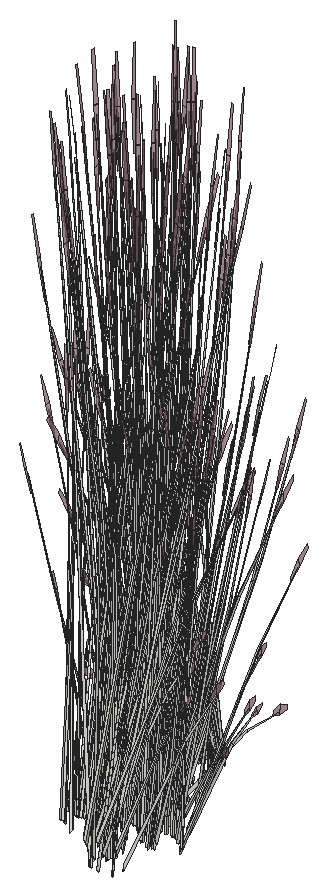
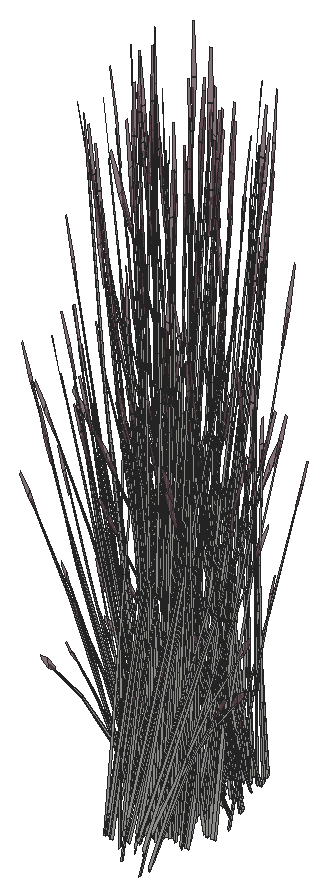
# SketchUp Ruby script. Lengths in inches.
U = 1.inch
M = Sketchup.active_model
def pt(a) = Geom::Point3d.new(a.map { |v| v * U })
def face(e, loops, mat)
  f = e.add_face(loops[0].map { |a| pt(a) })
  loops[1..].each { |l| e.add_face(l.map { |a| pt(a) }).erase! }
  f.material = f.back_material = mat if mat
  f
end
# faces: each face lists its corners as indices into pts; further lists are holes
def faces(e, pts, list, mat = nil) = list.each { |f| face(e, (f[0].is_a?(Array) ? f : [f]).map { |l| l.map { |i| pts[i] } }, mat) }
# xy, xz, yz: faces in a plane at the given z, y or x. An outline is a flat list of corners, or four numbers for a rectangle; further outlines are holes
def ring(l) = l.size == 4 ? [[l[0], l[1]], [l[2], l[1]], [l[2], l[3]], [l[0], l[3]]] : l.each_slice(2).to_a
def flat(e, list, mat, &to3) = list.each { |f| face(e, (f[0].is_a?(Array) ? f : [f]).map { |l| ring(l).map { |u, v| to3.(u, v) } }, mat) }
def xy(e, z, list, mat = nil) = flat(e, list, mat) { |x, y| [x, y, z] }
def xz(e, y, list, mat = nil) = flat(e, list, mat) { |x, z| [x, y, z] }
def yz(e, x, list, mat = nil) = flat(e, list, mat) { |y, z| [x, y, z] }
def lines(e, pts, list) = list.each { |a, b| e.add_line(pt(pts[a]), pt(pts[b])) }
# prism: a flat outline (further loops are holes) pulled along v
def prism(e, loops, v, mat = nil)
  f = face(e, loops, mat); d = Geom::Vector3d.new(v.map { |x| x * U })
  f.pushpull(f.normal.samedirection?(d) ? d.length : -d.length)
end
def box(e, o, s, mat = nil) = prism(e, [[o, [o[0] + s[0], o[1], o[2]], [o[0] + s[0], o[1] + s[1], o[2]], [o[0], o[1] + s[1], o[2]]]], [0, 0, s[2]], mat)
def at(x, y, z, deg = 0) = Geom::Transformation.translation(pt([x, y, z])) * Geom::Transformation.rotation(ORIGIN, Z_AXIS, deg.degrees)
def axes(o, x, y, z) = Geom::Transformation.new([*x, 0, *y, 0, *z, 0, *pt(o).to_a, 1])
def part(name) = M.definitions.add(name)
# library, detail: a bought-in or finely detailed component or shape, given as its bounding box
def library(name, o, s) = part(name).tap { |d| box(d.entities, o, s) }
def detail(e, o, s) = box(e.add_group.entities, o, s)
def put(e, d, t, mat = nil) = e.add_instance(d, t).tap { |i| i.material = mat if mat }
def group(e, t, mat = nil) = e.add_group.tap { |g| g.transformation = t; g.material = mat if mat }.entities
root = M.entities
M.materials.add("LightPink_Translucent").color = [144, 107, 117]
M.materials["LightPink_Translucent"].alpha = 0.75
c1 = part("blade")
p = [[2.15,0.21,22],[0,0.17,0],[0.09,0.45,0],[2.18,0.31,22],[2.29,0.31,22],[0.38,0.45,0],
  [2.48,0.24,33],[2.49,0.24,33],[2.48,0.22,33]]
faces(c1.entities,p,[[0,1,2,3],[4,5,2,3],[6,3,4,7],[8,0,3,6]])
c2 = part("seeds")
p = [[0.3,-0.1,1.38],[-0.01,-0.03,1.59],[-0.01,-0.03,0.03],[0.14,-0.07,-0.07],[0.29,-0.03,3],[0.15,0.01,3.11]]
faces(c2.entities,p,[[0,1,2,3],[1,0,4,5]],"LightPink_Translucent")
c3 = part("blade with seeds")
put(c3.entities,c1,at(0,0,0))
put(c3.entities,c2,axes([2.4,0.25,30.99],[1.5799,-0.05474,1.17369],[-0.12525,1.92788,0.29478],[-0.07173,-0.02425,1.56792]))
put(root,c3,axes([411.74,290.53,-9.94],[-0.24813,0.48978,-0.41661],[-0.51557,-0.23571,0.2005],[0,0.1129,1.33761]))
put(root,c3,axes([412.8,291.68,-7.59],[-0.37709,0.35815,0.447],[-0.32522,-0.38035,0.36857],[0.17692,0.06607,0.92496]))
put(root,c3,axes([411.27,295.7,-10.08],[0.34446,-0.40855,-0.58063],[0.42791,0.37046,-0.15239],[0.13803,-0.10191,1.28164]))
put(root,c3,axes([413.76,294.73,-9.42],[-0.17034,0.27669,1.06958],[-0.14642,-0.37174,0.78586],[0.14069,-0.09315,0.23558]))
put(root,c3,axes([413.51,295.77,-7.78],[0.44516,-0.07768,-0.32977],[0.11755,0.44407,0.42575],[0.12757,-0.11927,0.81462]))
put(root,c3,axes([407.94,292.07,-6.74],[0.45129,0.14509,-0.06041],[-0.13882,0.44656,-0.27392],[-0.07381,0.0678,0.90349]))
put(root,c3,axes([411.14,291.24,-10.08],[-0.34446,0.40855,-0.58063],[-0.42791,-0.37046,-0.15239],[-0.13803,0.10191,1.28164]))
put(root,c3,axes([409.34,295.03,-7.6],[0.02575,-0.41332,0.05988],[0.38885,0.01133,0.47138],[-0.14895,-0.04325,0.71878]))
put(root,c3,axes([411.6,292.1,-7.3],[-0.07899,-0.43781,0.32977],[0.45153,-0.11561,-0.42575],[0.12128,0.12546,0.81462]))
put(root,c3,axes([410.67,296.42,-9.94],[0.24813,-0.48978,-0.41661],[0.51557,0.23571,0.2005],[0,-0.1129,1.33761]))
put(root,c3,axes([411.76,291.93,-9.83],[0.64025,0.17667,0.2864],[-0.16018,0.63149,-0.33981],[-0.10597,0.07904,1.53541]))
put(root,c3,axes([411.71,292.36,-10.12],[-0.47863,0.27177,-0.46235],[-0.28609,-0.48733,0],[-0.10901,0.0619,1.46668]))
put(root,c3,axes([413.3,290.75,-10.12],[0,0.54355,-0.46235],[-0.57217,0,0],[0,0.1238,1.46668]))
put(root,c3,axes([410.9,296.17,-9.52],[-0.05959,-0.62022,-0.27094],[0.62068,-0.0375,-0.46562],[0.1093,-0.08261,1.4872]))
put(root,c3,axes([411.87,290.81,-8.39],[-0.18996,-0.09365,1.59586],[0.39312,-0.39287,0.12904],[0.24502,0.17723,0.68222]))
put(root,c3,axes([409.36,296.21,-10.11],[0.35699,-0.33913,-0.28847],[0.35699,0.33913,0.28847],[0,-0.10923,1.29413]))
put(root,c3,axes([411.91,289.58,-7.83],[-0.44191,-0.28242,1.28769],[0.46662,-0.43971,0.5556],[0.14258,0.26499,1.24467]))
put(root,c3,axes([409.22,294.58,-10.02],[-0.14753,0.44383,-0.03625],[-0.45406,-0.13653,-0.16435],[-0.06894,-0.07259,0.54209]))
put(root,c3,axes([413.15,296.03,-7.3],[-0.44516,0.07768,0.32977],[-0.11755,-0.44407,-0.42575],[0.12757,-0.11927,0.81462]))
put(root,c3,axes([410.61,296.82,-9.52],[-0.57594,-0.25935,-0.27094],[0.27732,-0.5474,-0.46562],[-0.0181,-0.1344,1.4872]))
put(root,c3,axes([408.97,296.61,-9.79],[-0.63949,0,0],[0,-0.60749,-0.48057],[0,-0.13836,1.52448]))
put(root,c3,axes([408.72,290.77,-7.3125],[0.47307,0.29971,-0.11324],[-0.27254,0.43404,-0.62851],[-0.13365,0.15087,0.95501]))
put(root,c3,axes([412.57,291.875,-9.42],[-0.28795,-0.15629,1.06958],[0.37181,-0.1588,0.78586],[0.10029,0.13452,0.23558]))
put(root,c3,axes([411.5625,292.32,-7.3125],[0.30474,-0.46525,-0.11324],[0.44133,0.26804,-0.62851],[0.15341,0.13145,0.95501]))
put(root,c3,axes([410.82,294.8,-10.11],[0.47712,0.13449,-0.28847],[-0.12013,0.47362,0.28847],[0.09619,-0.05462,1.29413]))
put(root,c3,axes([408.95,291.125,-7.64],[0.13138,0.49631,-0.47583],[-0.49754,0.08682,-0.36857],[-0.14258,0.13331,0.91046]))
put(root,c3,axes([409.55,291.69,-7.3],[0.34603,-0.28618,0.32977],[0.32756,0.32677,-0.42575],[-0.04984,0.16603,0.81462]))
put(root,c3,axes([412.14,292.27,-9.79],[0.31974,0.54466,0],[-0.53494,0.30375,-0.48057],[-0.12184,0.06918,1.52448]))
put(root,c3,axes([411.16,292.71,-7.62],[0.00151,-0.06581,1.65179],[0.43826,-0.29033,-0.15608],[0.15223,0.10363,0.29231]))
put(root,c3,axes([413.55,295.96,-7.6],[0.35109,0.22859,0.05988],[-0.2044,0.32553,0.47138],[0.11256,-0.10524,0.71878]))
put(root,c3,axes([412.65,292.46,-10.61],[0.03726,-0.07847,1.6421],[0.46909,-0.23111,-0.25086],[0.14221,0.11962,0.2797]))
put(root,c3,axes([413.46,295.87,-7.59],[0.12683,0.50025,0.447],[-0.49754,0.08682,0.36857],[0.14663,-0.11765,0.92496]))
put(root,c3,axes([411.87,290.12,-9.35],[-0.01397,-0.51177,1.31553],[0.63227,0.13266,0.557],[-0.14954,0.28003,1.24175]))
put(root,c3,axes([412.03,290.67,-10.05],[0.18752,0.49766,-0.6445],[-0.54017,0.17923,-0.16915],[0.02073,0.16852,1.42262]))
put(root,c3,axes([409.24,291.95,-7.6],[-0.42027,-0.02533,0.05988],[0.01152,-0.38243,0.47138],[-0.04398,0.14649,0.71878]))
put(root,c3,axes([414.8,296.47,-7.61],[0.07097,-0.08279,1.62908],[-0.09083,-0.50786,-0.25764],[0.17806,-0.09629,0.13065]))
put(root,c3,axes([409.37,291.99,-7.59],[-0.36417,-0.37086,0.447],[0.38674,-0.31985,0.36857],[-0.06718,0.174,0.92496]))
put(root,c3,axes([411.92,292.09,-7.64],[0.50465,-0.12921,-0.47583],[0.08828,0.48932,-0.36857],[0.13555,0.14022,0.91046]))
put(root,c3,axes([410.52,292.16,-7.3],[0.15418,-0.41799,0.32977],[0.44981,0.12192,-0.42575],[0.04124,0.16829,0.81462]))
put(root,c3,axes([409.47,296.45,-9.83],[-0.47569,0.45698,0.2864],[-0.47598,-0.45217,-0.33981],[-0.01661,-0.12977,1.53541]))
put(root,c3,axes([412.62,292.59,-9.52],[-0.32795,-0.01705,0.97832],[0.21658,-0.36206,0.54015],[0.12956,0.12863,0.76741]))
put(root,c3,axes([410.98,296.66,-9.73],[0.57623,0.26344,0.22409],[-0.27732,0.5474,0.46562],[0,-0.12618,1.49497]))
put(root,c3,axes([410.76,297.4,-9.73],[0.13555,-0.64407,-0.21817],[0.64269,0.11227,0.47743],[-0.1123,-0.08895,1.45677]))
put(root,c3,axes([411.67,292.49,-7.6],[-0.23243,0.34529,0.05988],[-0.331,-0.20103,0.47138],[0.10701,0.1107,0.71878]))
put(root,c3,axes([409.6,295.34,-7.3],[0.29098,0.34031,0.32977],[-0.33226,0.32215,-0.42575],[-0.16881,-0.04902,0.81462]))
put(root,c3,axes([411.13,293.66,-6.74],[0.35341,-0.31182,-0.06041],[0.32382,0.34152,-0.27392],[0.0228,0.09677,0.90349]))
put(root,c3,axes([411.77,292.4,-7.59],[-0.50866,0.12474,0.447],[-0.08828,-0.48932,0.36857],[0.11963,0.14421,0.92496]))
put(root,c3,axes([410.79,296.29,-9.47],[-0.55535,0.03355,0.41661],[-0.05022,-0.55698,-0.2005],[0.09942,-0.05645,1.33761]))
put(root,c3,axes([409.26,291.05,-8.39],[0.09522,-0.18683,1.59586],[0.39947,0.38663,0.12904],[-0.18021,0.24097,0.68222]))
put(root,c3,axes([409.36,296.7,-9.69],[0,0.54355,0.46235],[-0.57217,0,0],[0,-0.1238,1.46668]))
put(root,c3,axes([413.4,297.24,-7.3125],[-0.25732,-0.49218,-0.11324],[0.45669,-0.24187,-0.62851],[0.19245,-0.06494,0.95501]))
put(root,c3,axes([411.55,291.71,-9.59],[0.00902,-0.18018,1.33163],[0.43127,-0.20126,-0.28638],[0.13313,0.21566,0.56934]))
put(root,c3,axes([413.38,296.82,-7.64],[0.13855,-0.49442,-0.47583],[0.47502,0.16947,-0.36857],[0.19125,-0.04534,0.91046]))
put(root,c3,axes([412.625,294.81,-9.79],[0.31974,-0.54466,0],[0.53494,0.30375,-0.48057],[0.12184,0.06918,1.52448]))
put(root,c3,axes([410.71,297.14,-9.94],[-0.30722,-0.45622,-0.41661],[0.46535,-0.32126,0.2005],[-0.09942,-0.05645,1.33761]))
put(root,c3,axes([410.78,296.49,-9.8],[0.22235,0.6078,0.42607],[-0.63531,0.21135,0.16719],[0.00776,-0.11168,1.47927]))
put(root,c3,axes([410.38,292.54,-7.6],[-0.37684,0.18473,0.05988],[-0.18445,-0.33686,0.47138],[0.03639,0.14849,0.71878]))
put(root,c3,axes([409.37,292.1,-7.78],[-0.34603,0.28618,-0.32977],[-0.32756,-0.32677,0.42575],[-0.04984,0.16603,0.81462]))
put(root,c3,axes([408.18,292.02,-7.61],[-0.01271,0.10756,1.62908],[0.36076,0.37419,-0.25764],[-0.09444,0.17695,0.13065]))
put(root,c3,axes([409.33,291.77,-6.97],[0.56206,0.02693,-0.12569],[-0.01536,0.50991,-0.69765],[-0.03904,0.19638,1.06006]))
put(root,c3,axes([410.37,292.34,-7.3125],[0.50045,-0.25306,-0.11324],[0.24593,0.44915,-0.62851],[0.06603,0.18927,0.95501]))
put(root,c3,axes([413.88,296.96,-10.15],[-0.32938,0.06523,1.31842],[-0.05243,-0.51922,0.07547],[0.2307,-0.07859,0.75023]))
put(root,c3,axes([414.48,296.5,-9.89],[-0.31706,-0.34757,-0.06041],[0.34725,-0.31847,-0.27392],[0.09839,-0.02242,0.90349]))
put(root,c3,axes([410.52,292.51,-7.28],[-0.50393,-0.1421,0.49617],[0.17232,-0.46717,0.40911],[0.03028,0.18372,1.0267]))
put(root,c3,axes([409.59,293.21,-9.42],[-0.01324,-0.32319,1.06958],[0.33072,0.23052,0.78586],[-0.06504,0.15405,0.23558]))
put(root,c3,axes([410.66,296.97,-9.47],[-0.24813,0.48978,0.41661],[-0.51557,-0.23571,-0.2005],[0,-0.1129,1.33761]))
put(root,c3,axes([411.58,296.55,-9.95],[0,-0.62892,0],[0.63949,0,0],[0,0,1.6711]))
put(root,c3,axes([412.35,295.09,-9.69],[-0.47863,-0.27177,0.46235],[0.28609,-0.48733,0],[0.10901,0.0619,1.46668]))
put(root,c3,axes([413.29,297,-7.36],[0.44939,-0.24006,-0.66157],[0.25044,0.49415,0.07984],[0.21713,-0.05613,0.93586]))
put(root,c3,axes([410.46,292.4375,-10.61],[0.08277,-0.02958,1.6421],[0.49786,0.16279,-0.25086],[0.01456,0.18348,0.2797]))
put(root,c3,axes([410.4375,297.3125,-10.08],[-0.53199,-0.08911,-0.58063],[0.11226,-0.54969,-0.15239],[-0.15876,-0.06661,1.28164]))
put(root,c3,axes([411.27,296.15,-9.8],[-0.42403,0.49328,0.42607],[-0.50377,-0.43543,0.16719],[0.10223,-0.04923,1.47927]))
put(root,c3,axes([409.72,291.96,-7.34],[0.3661,0.36521,-0.52818],[-0.38674,0.31985,-0.40911],[-0.0557,0.18556,1.01061]))
put(root,c3,axes([411.74,297.03,-9.86],[-0.47569,-0.46784,-0.05709],[0.47598,-0.46812,0],[-0.01661,-0.01634,1.63492]))
put(root,c3,axes([409.32,292.51,-9.37],[0.46459,-0.09625,0.0606],[0.10681,0.38778,-0.80367],[-0.02945,0.1963,0.72038]))
put(root,c3,axes([410.8,292.32,-7.64],[0.50273,0.13626,-0.47583],[-0.17232,0.46717,-0.36857],[0.0461,0.18809,0.91046]))
put(root,c3,axes([411.09,291.35,-8.39],[-0.1169,-0.17452,1.59586],[0.54019,-0.14692,0.12904],[0.12209,0.27397,0.68222]))
put(root,c3,axes([410.54,295.34,-9.7],[-0.14774,0.54019,0.16428],[-0.54062,-0.15287,0.32672],[0.09339,-0.00263,1.49371]))
put(root,c3,axes([413.22,297.09,-7.3],[-0.42502,-0.15163,0.32977],[0.12396,-0.44238,-0.42575],[0.17112,-0.04056,0.81462]))
put(root,c3,axes([410.3125,295.77,-10.52],[-0.50338,0.21762,1.20058],[-0.16022,-0.62439,0.4665],[0.30911,0.01039,1.36553]))
put(root,c3,axes([411.67,295.9375,-9.5625],[0.09866,-0.48509,0.13483],[0.48202,0.0842,-0.38503],[0.08772,0.04981,1.18024]))
put(root,c3,axes([410.57,292.61,-7.78],[-0.15418,0.41799,-0.32977],[-0.44981,-0.12192,0.42575],[0.04124,0.16829,0.81462]))
put(root,c3,axes([410.83,297.09,-9.8],[0.64638,0.11452,0.42607],[-0.13155,0.64678,0.16719],[-0.09446,-0.06245,1.47927]))
put(root,c3,axes([414.24,296.62,-10.61],[-0.02673,-0.08252,1.6421],[0.18538,-0.48271,-0.25086],[0.187,-0.00694,0.2797]))
put(root,c3,axes([411.46,296.06,-9.47],[-0.30722,-0.45622,0.41661],[0.46535,-0.32126,-0.2005],[0.09942,0.05645,1.33761]))
put(root,c3,axes([409.6,291.8,-7.03],[-0.01331,0.50278,-0.73435],[-0.56035,-0.03377,0.08862],[-0.05914,0.213,1.03881]))
put(root,c3,axes([408.14,293.12,-7.62],[0.05802,-0.03282,1.65179],[0.47954,0.21828,-0.15608],[-0.01127,0.18175,0.29231]))
put(root,c3,axes([409.87,298.15,-10.11],[-0.12013,-0.47362,-0.28847],[0.47712,-0.13449,0.28847],[-0.09619,-0.05462,1.29413]))
put(root,c3,axes([410.13,291.44,-8.39],[-0.01252,-0.20862,1.59586],[0.54251,0.1384,0.12904],[-0.03356,0.2973,0.68222]))
put(root,c3,axes([410.48,298.12,-9.7],[0.54955,-0.14427,0.16428],[0.1357,0.53689,0.32672],[-0.04901,-0.07823,1.49371]))
put(root,c3,axes([411.62,296.09,-9.52],[0.51635,-0.36087,-0.27094],[0.34336,0.5099,-0.46562],[0.1274,0.05178,1.4872]))
put(root,c3,axes([413.67,297.05,-7.78],[0.42502,0.15163,-0.32977],[-0.12396,0.44238,0.42575],[0.17112,-0.04056,0.81462]))
put(root,c3,axes([409.74,298.35,-10.12],[-0.47863,-0.27177,-0.46235],[0.28609,-0.48733,0],[-0.10901,-0.0619,1.46668]))
put(root,c3,axes([412.92,295.14,-10.12],[0.47863,0.27177,-0.46235],[-0.28609,0.48733,0],[0.10901,0.0619,1.46668]))
put(root,c3,axes([410.62,292.23,-7.36],[0.24409,0.44196,-0.66157],[-0.50245,0.2463,0.07984],[0.05708,0.21354,0.93586]))
put(root,c3,axes([412.01,296.6875,-9.95],[0.57217,0,0],[0,0.56272,0],[0,0,1.66132]))
put(root,c3,axes([411.04,297.39,-9.52],[-0.51635,0.36087,-0.27094],[-0.34336,-0.5099,-0.46562],[-0.1274,-0.05178,1.4872]))
put(root,c3,axes([412.17,295.37,-9.7],[-0.54955,0.14427,0.16428],[-0.1357,-0.53689,0.32672],[0.04901,0.07823,1.49371]))
put(root,c3,axes([409.21,292.93,-9.59],[0.16138,-0.08575,1.33163],[0.39845,0.25854,-0.28638],[-0.1186,0.22371,0.56934]))
put(root,c3,axes([410.25,293.35,-7.61],[0.06483,0.08753,1.62908],[0.52315,0.03439,-0.25764],[0.05261,0.19303,0.13065]))
put(root,c3,axes([412.51,296.5,-8.39],[-0.21212,0.01231,1.59586],[0.14072,-0.53355,0.12904],[0.3023,0.033,0.68222]))
put(root,c3,axes([412.78,295.34,-10.11],[0.12013,0.47362,-0.28847],[-0.47712,0.13449,0.28847],[0.09619,0.05462,1.29413]))
put(root,c3,axes([413.61,297.23,-7.6],[0.18783,0.37061,0.05988],[-0.34252,0.1814,0.47138],[0.15099,-0.03579,0.71878]))
put(root,c3,axes([411.82,296.4,-9.78],[-0.64638,-0.11452,0.45814],[0.13155,-0.64678,0.17978],[0.09446,0.06245,1.59061]))
put(root,c3,axes([413.57,297.1,-7.59],[-0.14449,0.4956,0.447],[-0.47502,-0.16947,0.36857],[0.1868,-0.02978,0.92496]))
put(root,c3,axes([411.31,298,-9.95],[-0.16686,-0.46861,0],[0.47648,-0.16411,0],[0,0,1.4375]))
put(root,c3,axes([410.99,297.55,-9.5625],[-0.09866,0.48509,0.13483],[-0.48202,-0.0842,-0.38503],[-0.08772,-0.04981,1.18024]))
put(root,c3,axes([409.12,296.29,-7.3],[0.42502,0.15163,0.32977],[-0.12396,0.44238,-0.42575],[-0.17112,0.04056,0.81462]))
put(root,c3,axes([411.93,297.93,-9.97],[0.53691,-0.18442,-0.17877],[0.18866,0.53125,0.00007],[0.05927,-0.02038,1.61933]))
put(root,c3,axes([412.12,298.15,-9.7],[0.14774,-0.54019,0.16428],[0.54062,0.15287,0.32672],[-0.09339,0.00263,1.49371]))
put(root,c3,axes([412,296.93,-9.9375],[0.35699,0.35109,0],[-0.35699,0.35109,0],[0,0,1.57621]))
put(root,c3,axes([409.41,292.51,-8.87],[0.01124,-0.2806,1.43727],[0.50537,0.14821,0.19862],[-0.04379,0.29905,0.67868]))
put(root,c3,axes([412.96,296.77,-9.7],[-0.40181,-0.39593,0.16428],[0.40492,-0.38402,0.32672],[-0.04438,0.08086,1.49371]))
put(root,c3,axes([412.22,296.18,-10.08],[0.53199,0.08911,-0.58063],[-0.11226,0.54969,-0.15239],[0.15876,0.06661,1.28164]))
put(root,c3,axes([414.57,297.14,-9.42],[-0.31598,0.08973,1.06958],[0.14873,-0.37085,0.78586],[0.16763,0.02538,0.23558]))
put(root,c3,axes([411.19,298.21,-9.95],[-0.51557,-0.24403,0],[0.24813,-0.50705,0],[0,0,1.51513]))
put(root,c3,axes([411.62,297.56,-9.7],[-0.49938,-0.43748,-0.23459],[0.42021,-0.49126,0.51337],[-0.13447,0.05118,1.56642]))
put(root,c3,axes([410.31,298.4,-9.69],[0.47863,0.27177,0.46235],[-0.28609,0.48733,0],[-0.10901,-0.0619,1.46668]))
put(root,c3,axes([411.99,296.52,-9.47],[0.24813,-0.48978,0.41661],[0.51557,0.23571,-0.2005],[0,0.1129,1.33761]))
put(root,c3,axes([414.42,298.71,-7.62],[-0.04624,-0.04758,1.65179],[0.10116,-0.51007,-0.15608],[0.18215,-0.03259,0.29231]))
put(root,c3,axes([411.9,296.8,-9.87],[0,0.62861,-0.05249],[-0.63949,0,0],[0,0.01975,1.67027]))
put(root,c3,axes([411.94,296.35,-9.94],[0.30722,0.45622,-0.41661],[-0.46535,0.32126,0.2005],[0.09942,0.05645,1.33761]))
put(root,c3,axes([414.02,298.28,-8.34],[-0.09788,-0.45691,-0.03251],[0.46264,-0.10504,-0.14742],[0.09661,0.02897,0.48626]))
put(root,c3,axes([410.03,298.68,-9.79],[-0.31974,0.54466,0],[-0.53494,-0.30375,-0.48057],[-0.12184,-0.06918,1.52448]))
put(root,c3,axes([412.82,298.27,-7.3125],[0.02738,-0.55277,-0.11324],[0.51847,0.01511,-0.62851],[0.19968,0.0384,0.95501]))
put(root,c3,axes([413.29,296.79,-9.69],[0,-0.54355,0.46235],[0.57217,0,0],[0,0.1238,1.46668]))
put(root,c3,axes([411.86,297.2,-9.47],[0.55535,-0.03355,0.41661],[0.05022,0.55698,-0.2005],[-0.09942,0.05645,1.33761]))
put(root,c3,axes([412.21,296.63,-9.5625],[0.47648,-0.15851,0.13483],[0.16686,0.45265,-0.38503],[0,0.09962,1.18024]))
put(root,c3,axes([412.74,298.05,-7.3],[-0.29098,-0.34031,0.32977],[0.33226,-0.32215,-0.42575],[0.16881,0.04902,0.81462]))
put(root,c3,axes([411.37,297.47,-9.94],[-0.55535,0.03355,-0.41661],[-0.05022,-0.55698,0.2005],[-0.09942,0.05645,1.33761]))
put(root,c3,axes([413.98,297.73,-9.59],[-0.12317,-0.13368,1.33163],[0.16025,-0.44223,-0.28638],[0.24919,0.05991,0.56934]))
put(root,c3,axes([409.44,303.25,-8.39],[0.1169,0.17452,1.59586],[-0.54019,0.14692,0.12904],[-0.12209,-0.27397,0.68222]))
put(root,c3,axes([411.78,298.22,-9.95],[0.51557,0.24403,0],[-0.24813,0.50705,0],[0,0,1.62917]))
put(root,c3,axes([410.33,302.09,-7.61],[-0.07822,-0.07621,1.62908],[-0.52201,0.04832,-0.25764],[-0.08331,-0.18228,0.13065]))
put(root,c3,axes([411.54,302.99,-9.59],[-0.14537,0.11002,1.33163],[-0.43536,-0.19256,-0.28638],[0.0807,-0.23948,0.56934]))
put(root,c3,axes([410.88,303.38,-7.36],[-0.24409,-0.44196,-0.66157],[0.50245,-0.2463,0.07984],[-0.05708,-0.21354,0.93586]))
put(root,c3,axes([413.27,297.93,-7.61],[0.10971,-0.00919,1.62908],[0.30091,-0.42228,-0.25764],[0.19514,0.05574,0.13065]))
put(root,c3,axes([411.98,298.76,-9.96],[-0.31576,-0.54657,-0.04789],[0.53494,-0.30375,0.48057],[-0.13182,0.05204,1.52373]))
put(root,c3,axes([411.87,297.44,-9.5625],[0.37783,0.32657,0.13483],[-0.31516,0.36844,-0.38503],[-0.08772,0.04981,1.18024]))
put(root,c3,axes([409.29,302.79,-9.59],[-0.03097,0.17781,1.33163],[-0.45273,0.14885,-0.28638],[-0.10583,-0.22982,0.56934]))
put(root,c3,axes([408.79,297.42,-7.6],[-0.35109,-0.22859,0.05988],[0.2044,-0.32553,0.47138],[-0.11256,0.10524,0.71878]))
put(root,c3,axes([410.46,302.4,-10.61],[-0.08578,0.01958,1.6421],[-0.47437,-0.22044,-0.25086],[0.00796,-0.18387,0.2797]))
put(root,c3,axes([412.85,298,-7.36],[0.51122,0.01309,-0.66157],[-0.03434,0.5511,0.07984],[0.21658,0.05816,0.93586]))
put(root,c3,axes([411.9,303.81,-7.36],[0.01331,-0.50278,-0.66157],[0.56035,0.03377,0.07984],[0.05914,-0.213,0.93586]))
put(root,c3,axes([412.27,298.44,-9.69],[0.47863,-0.27177,0.46235],[0.28609,0.48733,0],[-0.10901,0.0619,1.46668]))
put(root,c3,axes([411.59,298.01,-9.87],[0.22235,0.62444,-0.05599],[-0.63531,0.21881,0],[0.00776,0.02181,1.60327]))
put(root,c3,axes([412.68,303.02,-7.61],[-0.00494,-0.10818,1.62908],[-0.41695,-0.31265,-0.25764],[0.06446,-0.18952,0.13065]))
put(root,c3,axes([410.93,303,-7.78],[0.15418,-0.41799,-0.32977],[0.44981,0.12192,0.42575],[-0.04124,-0.16829,0.81462]))
put(root,c3,axes([411.27,303.55,-8.39],[-0.09522,0.18683,1.59586],[-0.39947,-0.38663,0.12904],[0.18021,-0.24097,0.68222]))
put(root,c3,axes([411.84,298.6875,-10.11],[-0.47712,-0.13449,-0.28847],[0.12013,-0.47362,0.28847],[-0.09619,0.05462,1.29413]))
put(root,c3,axes([412.57,302.64,-7.62],[-0.05194,0.04152,1.65179],[-0.50886,-0.14007,-0.15608],[-0.01842,-0.18118,0.29231]))
put(root,c3,axes([409.19,297.35,-7.3],[0.44516,-0.07768,0.32977],[0.11755,0.44407,-0.42575],[-0.12757,0.11927,0.81462]))
put(root,c3,axes([413.68,296.88,-9.79],[0.63949,0,0],[0,0.60749,-0.48057],[0,0.13836,1.52448]))
put(root,c3,axes([413.43,297.19,-9.95],[-0.63917,-0.00435,-0.04634],[0,-0.60749,0.46507],[-0.02009,0.13829,1.47457]))
put(root,c3,axes([412.04,296.66,-9.52],[0.57594,0.25935,-0.27094],[-0.27732,0.5474,-0.46562],[0.0181,0.1344,1.4872]))
put(root,c3,axes([410.7,303.29,-7.64],[-0.50273,-0.13626,-0.47583],[0.17232,-0.46717,-0.36857],[-0.0461,-0.18809,0.91046]))
put(root,c3,axes([411.01,302.12,-9.42],[0.06561,0.31695,1.06958],[-0.36394,-0.17555,0.78586],[0.03916,-0.16229,0.23558]))
put(root,c3,axes([413.15,298.23,-7.78],[0.29098,0.34031,-0.32977],[-0.33226,0.32215,0.42575],[0.16881,0.04902,0.81462]))
put(root,c3,axes([413.29,297.28,-10.11],[-0.35699,0.33913,-0.28847],[-0.35699,-0.33913,0.28847],[0,0.10923,1.29413]))
put(root,c3,axes([411.78,303.64,-7.64],[-0.3661,-0.36521,-0.47583],[0.38674,-0.31985,-0.36857],[0.0557,-0.18556,0.91046]))
put(root,c3,axes([411.76,297.31,-9.52],[0.05959,0.62022,-0.27094],[-0.62068,0.0375,-0.46562],[-0.1093,0.08261,1.4872]))
put(root,c3,axes([413.01,298.36,-7.6],[-0.02575,0.41332,0.05988],[-0.38885,-0.01133,0.47138],[0.14895,0.04325,0.71878]))
put(root,c3,axes([411.98,297.07,-9.94],[-0.24813,0.48978,-0.41661],[-0.51557,-0.23571,0.2005],[0,0.1129,1.33761]))
put(root,c3,axes([409.8,301.84,-7.62],[-0.00954,0.06515,1.65179],[-0.47055,0.23645,-0.15608],[-0.13847,-0.12087,0.29231]))
put(root,c3,axes([413.04,298.23,-7.59],[-0.37709,0.35815,0.447],[-0.32522,-0.38035,0.36857],[0.17692,0.06607,0.92496]))
put(root,c3,axes([409.69,303,-7.26],[0.56969,-0.13971,0.50064],[0.09887,0.54803,0.4128],[-0.13398,-0.16152,1.03595]))
put(root,c3,axes([410.98,303.1,-7.59],[0.50393,0.1421,0.447],[-0.17232,0.46717,0.36857],[-0.03028,-0.18372,0.92496]))
put(root,c3,axes([411.125,303.27,-7.3125],[-0.50045,0.25306,-0.11324],[-0.24593,-0.44915,-0.62851],[-0.06603,-0.18927,0.95501]))
put(root,c3,axes([412.17,303.83,-7.3125],[-0.56206,-0.02693,-0.11324],[0.01536,-0.50991,-0.62851],[0.03904,-0.19638,0.95501]))
put(root,c3,axes([408.18,298.62,-6.74],[0.45129,0.14509,-0.06041],[-0.13882,0.44656,-0.27392],[-0.07381,0.0678,0.90349]))
put(root,c3,axes([411.38,297.79,-10.08],[-0.34446,0.40855,-0.58063],[-0.42791,-0.37046,-0.15239],[-0.13803,0.10191,1.28164]))
put(root,c3,axes([412.125,303.51,-7.78],[0.34603,-0.28618,-0.32977],[0.32756,0.32677,0.42575],[0.04984,-0.16603,0.81462]))
put(root,c3,axes([409.14,302.5,-9.42],[0.26677,0.18918,1.06958],[-0.38851,0.11372,0.78586],[-0.08313,-0.14539,0.23558]))
put(root,c3,axes([411.12,303.0625,-7.6],[0.37684,-0.18473,0.05988],[0.18445,0.33686,0.47138],[-0.03639,-0.14849,0.71878]))
put(root,c3,axes([409.78,303.5,-7.36],[-0.43608,-0.26272,-0.66157],[0.30991,-0.46038,0.07984],[-0.158,-0.15687,0.93586]))
put(root,c3,axes([409.63,303.15,-7.78],[-0.07899,-0.43781,-0.32977],[0.45153,-0.11561,0.42575],[-0.12128,-0.12546,0.81462]))
put(root,c3,axes([411.84,298.64,-7.3],[-0.07899,-0.43781,0.32977],[0.45153,-0.11561,-0.42575],[0.12128,0.12546,0.81462]))
put(root,c3,axes([412,298.48,-9.83],[0.64025,0.17667,0.2864],[-0.16018,0.63149,-0.33981],[-0.10597,0.07904,1.53541]))
put(root,c3,axes([411.95,298.9,-10.12],[-0.47863,0.27177,-0.46235],[-0.28609,-0.48733,0],[-0.10901,0.0619,1.46668]))
